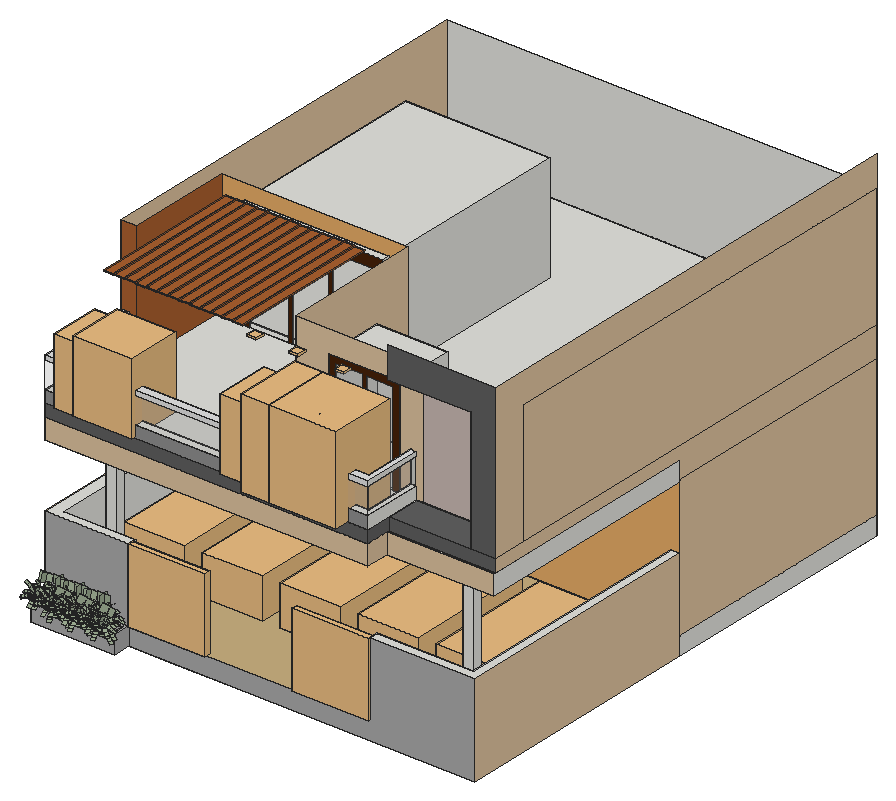
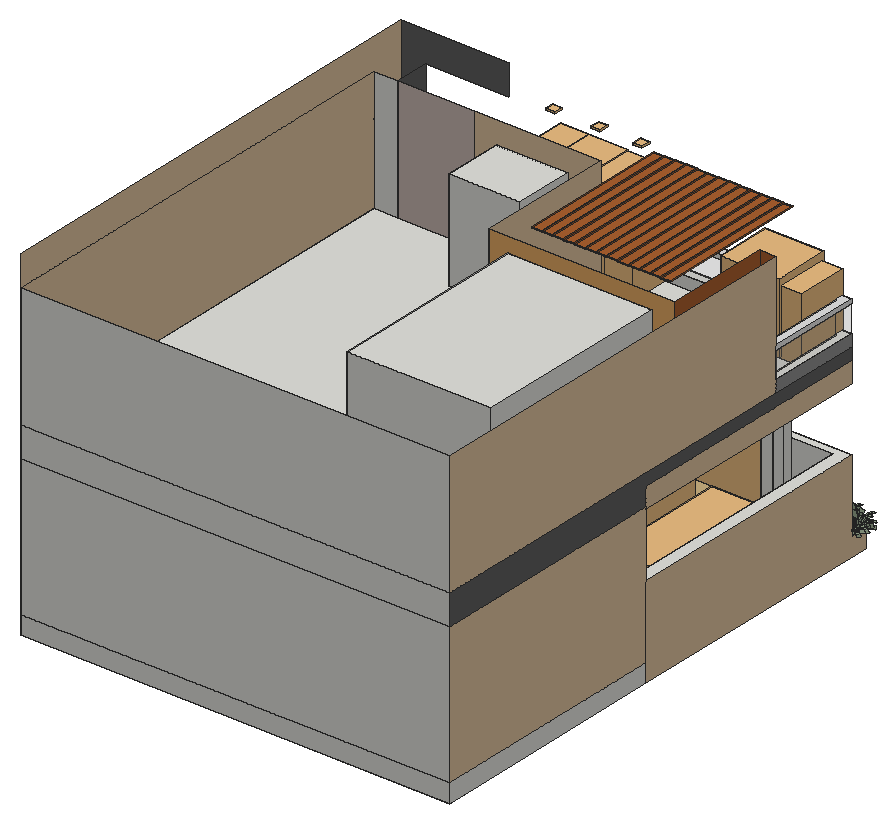
# SketchUp Ruby script. Lengths in inches.
U = 1.inch
M = Sketchup.active_model
def pt(a) = Geom::Point3d.new(a.map { |v| v * U })
def face(e, loops, mat)
  f = e.add_face(loops[0].map { |a| pt(a) })
  loops[1..].each { |l| e.add_face(l.map { |a| pt(a) }).erase! }
  f.material = f.back_material = mat if mat
  f
end
# faces: each face lists its corners as indices into pts; further lists are holes
def faces(e, pts, list, mat = nil) = list.each { |f| face(e, (f[0].is_a?(Array) ? f : [f]).map { |l| l.map { |i| pts[i] } }, mat) }
# xy, xz, yz: faces in a plane at the given z, y or x. An outline is a flat list of corners, or four numbers for a rectangle; further outlines are holes
def ring(l) = l.size == 4 ? [[l[0], l[1]], [l[2], l[1]], [l[2], l[3]], [l[0], l[3]]] : l.each_slice(2).to_a
def flat(e, list, mat, &to3) = list.each { |f| face(e, (f[0].is_a?(Array) ? f : [f]).map { |l| ring(l).map { |u, v| to3.(u, v) } }, mat) }
def xy(e, z, list, mat = nil) = flat(e, list, mat) { |x, y| [x, y, z] }
def xz(e, y, list, mat = nil) = flat(e, list, mat) { |x, z| [x, y, z] }
def yz(e, x, list, mat = nil) = flat(e, list, mat) { |y, z| [x, y, z] }
def lines(e, pts, list) = list.each { |a, b| e.add_line(pt(pts[a]), pt(pts[b])) }
# prism: a flat outline (further loops are holes) pulled along v
def prism(e, loops, v, mat = nil)
  f = face(e, loops, mat); d = Geom::Vector3d.new(v.map { |x| x * U })
  f.pushpull(f.normal.samedirection?(d) ? d.length : -d.length)
end
def box(e, o, s, mat = nil) = prism(e, [[o, [o[0] + s[0], o[1], o[2]], [o[0] + s[0], o[1] + s[1], o[2]], [o[0], o[1] + s[1], o[2]]]], [0, 0, s[2]], mat)
def at(x, y, z, deg = 0) = Geom::Transformation.translation(pt([x, y, z])) * Geom::Transformation.rotation(ORIGIN, Z_AXIS, deg.degrees)
def axes(o, x, y, z) = Geom::Transformation.new([*x, 0, *y, 0, *z, 0, *pt(o).to_a, 1])
def part(name) = M.definitions.add(name)
# library, detail: a bought-in or finely detailed component or shape, given as its bounding box
def library(name, o, s) = part(name).tap { |d| box(d.entities, o, s) }
def detail(e, o, s) = box(e.add_group.entities, o, s)
def put(e, d, t, mat = nil) = e.add_instance(d, t).tap { |i| i.material = mat if mat }
def group(e, t, mat = nil) = e.add_group.tap { |g| g.transformation = t; g.material = mat if mat }.entities
root = M.entities
M.materials.add("Generic").color = [222, 194, 159]
M.materials.add("Generic\#1").color = [230, 172, 103]
M.materials.add("Generic\#2").color = [241, 212, 157]
M.materials.add("[Color M01]").color = [226, 226, 226]
M.materials.add("[Color M03]").color = [170, 170, 170]
M.materials.add("[Color M04]").color = [142, 142, 142]
M.materials.add("[Color M07]").color = [96, 96, 96]
M.materials.add("[Roofing Slate Tan]").color = [200, 175, 128]
M.materials.add("[Stone Marble]").color = [201, 185, 179]
M.materials.add("[Translucent Glass Gray]").color = [175, 175, 175]
M.materials["[Translucent Glass Gray]"].alpha = 0.14
M.materials.add("[Wood Cherry Original]").color = [170, 96, 47]
M.materials.add("[Wood Veneer 01]").color = [71, 34, 9]
M.materials.add("hymenocallis littoralis").color = [156, 172, 146]
c1 = part("Group\#856")
xy(c1.entities,7.38,[[0,0,5.5,15.91]],"hymenocallis littoralis")
p = [[5.5,28.78,0],[5.5,26.79,3.44],[0,26.79,3.44],[0,28.78,0],[0,23.75,6],[5.5,23.75,6],
  [0,15.91,7.38],[5.5,15.91,7.38]]
faces(c1.entities,p,[[0,1,2,3],[4,2,1,5],[6,4,5,7]],"hymenocallis littoralis")
c2 = part("Group\#854")
xy(c2.entities,7.38,[[0,0,5.5,15.91],[0,15.91,5.5,23.87]],"hymenocallis littoralis")
p = [[5.5,31.07,4.3],[5.5,27.74,6.47],[0,27.74,6.47],[0,31.07,4.3],[0,23.87,7.38],[5.5,23.87,7.38]]
faces(c2.entities,p,[[0,1,2,3],[4,2,1,5]],"hymenocallis littoralis")
c3 = part("Group\#857")
xy(c3.entities,7.38,[[0,0,5.6,15.91]],"hymenocallis littoralis")
p = [[5.6,28.78,0],[5.6,26.79,3.44],[0,26.79,3.44],[0,28.78,0],[0,23.75,6],[5.6,23.75,6],
  [0,15.91,7.38],[5.6,15.91,7.38]]
faces(c3.entities,p,[[0,1,2,3],[4,2,1,5],[6,4,5,7]],"hymenocallis littoralis")
c4 = part("Group\#855")
put(c4.entities,c2,axes([6.09,8.57,-0.52],[0.446,0.85617,0.26089],[-0.18444,-0.19731,0.96283],[0.87582,-0.47754,0.0699]))
put(c4.entities,c2,axes([6.29,7.28,-1.71],[0.37058,0.92707,-0.05667],[-0.32382,0.19004,0.99128],[0.87712,-0.32925,0.34964]))
put(c4.entities,c2,axes([11.04,16.14,-0.7],[1,0,0],[0,0.16628,1.02662],[0,-1.18456,0.19186]))
c5 = part("Group\#860")
put(c5.entities,c1,axes([24.57,32.05,-1.76],[0.9552,-0.22102,-0.19681],[0.4036,0.95545,0.88585],[-0.00568,-0.67859,0.7345]))
put(c5.entities,c1,axes([23.95,29.24,-2.4],[0,1,0],[-0.76041,0,0.64945],[0.64945,0,0.76041]))
put(c5.entities,c1,axes([24.22,24.72,-0.48],[-0.70711,0.70711,0],[-0.32757,-0.32757,0.80237],[0.61237,0.61237,0.5]))
put(c5.entities,c2,axes([20.66,37.22,-0.63],[1.12361,0.03262,0.39091],[-0.43499,0.29739,0.78777],[0.09852,-1.27434,0.37535]))
put(c5.entities,c1,axes([28.75,24.45,-2.4],[-1,0,0],[0,-0.76041,0.64945],[0,0.64945,0.76041]))
put(c5.entities,c3,axes([30.4,30.98,-3.7],[0.65676,-0.72002,0.22414],[0.55667,0.66341,0.5],[-0.50871,-0.20361,0.83652]))
put(c5.entities,c3,axes([32.41,29.61,-3.7],[0.04029,-0.97372,0.22414],[0.85287,0.15038,0.5],[-0.52057,0.17102,0.83652]))
put(c5.entities,c1,axes([31.89,25.85,-1.76],[-0.92056,0.33739,-0.19681],[-0.5186,-0.89824,0.88585],[0.08952,0.67268,0.7345]))
put(c5.entities,c1,axes([25.55,34.78,-0.48],[0.86603,0.5,0],[-0.25,0.43301,0.86603],[0.43301,-0.75,0.5]))
put(c5.entities,c3,axes([20.4,16.9375,-8.07],[-0.70711,0.70711,0],[-0.35754,-0.35754,0.65422],[1.3987,1.3987,1.52882]))
put(c5.entities,c1,axes([32.86,34.14,-0.48],[0.76604,-0.64279,0],[0.32139,0.38302,0.86603],[-0.55667,-0.66341,0.5]))
put(c5.entities,c1,axes([27.15,34.7,-0.1],[0.82472,-0.17528,-0.53769],[0.53769,0.53769,0.64945],[0.17528,-0.82472,0.53769]))
put(c5.entities,c1,axes([33.58,28.77,-2.4],[0,-1,0],[0.76041,0,0.64945],[-0.64945,0,0.76041]))
put(c5.entities,c1,axes([26.43,23.87,-2.81],[-0.75126,0.04415,0.65853],[0.53769,-0.53769,0.64945],[0.38276,0.84199,0.3802]))
put(c5.entities,c1,axes([28.78,23.98,-2.4],[-1,0,0],[0,-0.76041,0.64945],[0,0.64945,0.76041]))
put(c5.entities,c1,axes([25.39,25.38,-2.4],[-0.70711,0.70711,0],[-0.53769,-0.53769,0.64945],[0.45923,0.45923,0.76041]))
put(c5.entities,c1,axes([27.32,21.63,-0.1],[-0.45923,0.70711,-0.53769],[-0.76041,0,0.64945],[0.45923,0.70711,0.53769]))
put(c5.entities,c1,axes([25.17,27.625,-1.76],[0.56416,0.80187,-0.19681],[-0.66673,0.66673,0.80532],[0.62659,-0.26057,0.7345]))
put(c5.entities,c3,axes([27.59,27.04,-3.96],[-0.8993,-0.06127,0.43301],[0.2962,-0.8138,0.5],[0.32175,0.57791,0.75]))
put(c5.entities,c3,axes([26.98,24.5,-3.18],[-0.5,0.86603,0],[-0.75,-0.43301,0.5],[0.43301,0.25,0.86603]))
put(c5.entities,c3,axes([24.55,27.74,-3.7],[0.29517,0.92878,0.22414],[-0.85287,0.15038,0.5],[0.43068,-0.33875,0.83652]))
put(c5.entities,c3,axes([24.26,29.8,-3.18],[0.76604,0.64279,0],[-0.47317,0.5639,0.425],[0.32139,-0.38302,0.86603]))
put(c5.entities,c3,axes([25.98,32.46,-3.18],[1,0,0],[0,0.86603,0.5],[0,-0.5,0.86603]))
put(c5.entities,c1,axes([28.78,33.57,-2.4],[1,0,0],[0,0.76041,0.64945],[0,-0.64945,0.76041]))
put(c5.entities,c4,at(14.99,21.38,2.5))
put(c5.entities,c2,axes([34.63,26.34,-1.46],[-0.70089,-0.70877,0.07994],[0.4756,-0.38088,0.79293],[-0.53156,0.59378,0.60405]))
put(c5.entities,c2,axes([28.14,16.92,1.8125],[-1.19719,0.6912,0],[-0.09607,-0.16641,0.94244],[0.68444,1.18549,0.17613]))
put(c5.entities,c2,axes([31.5625,35.84,0.97],[0.66765,-1.1564,0.35779],[0.04445,0.30732,0.91033],[-1.20828,-0.64496,0.17012]))
put(c5.entities,c2,axes([38.94,22.51,0.89],[-0.97932,-0.67164,-0.05202],[0.27787,-0.41401,0.90999],[-0.85985,0.93577,0.32097]))
put(c5.entities,c2,axes([38.44,21.09,1.98],[-1.02864,-0.54856,0.2395],[0.33481,0.06999,0.88388],[-0.77261,1.08328,0.06417]))
put(c5.entities,c3,axes([35.02,30.51,-1.3],[-0.17365,-0.98481,0],[0.60224,-0.10619,0.79122],[-0.7792,0.13739,0.61153]))
put(c5.entities,c3,axes([29.41,22.33,-1.3],[-0.93969,0.34202,0],[-0.20915,-0.57465,0.79122],[0.27061,0.74351,0.61153]))
put(c5.entities,c2,axes([19.64,36,-1.62],[1.18194,0.09546,0.08234],[-0.14377,0.68823,0.76313],[0.21457,-1.1326,0.62386]))
put(c5.entities,c3,axes([24.25,24.14,-1.3],[-0.34202,0.93969,0],[-0.57465,-0.20915,0.79122],[0.74351,0.27061,0.61153]))
put(c5.entities,c3,axes([25.98,34.61,-1.3],[1,0,0],[0,0.61153,0.79122],[0,-0.79122,0.61153]))
put(c5.entities,c3,axes([31.16,34.41,-1.64],[0.56518,-0.80224,-0.19234],[0.73413,0.34233,0.72935],[-0.47639,-0.50772,0.71782]))
put(c5.entities,c3,axes([40.52,26.84,-5.82],[-0.42262,-0.90631,0],[0.48019,-0.22391,0.68552],[-1.43418,0.66877,1.22305]))
put(c5.entities,c1,axes([29.86,38.42,-1.01],[0.89064,-0.37013,0.26413],[-0.03924,0.63286,1.01918],[-0.45353,-0.76487,0.45748]))
put(c5.entities,c1,axes([29.34,22.4,-0.48],[-0.99619,-0.08716,0],[0.04358,-0.4981,0.86603],[-0.07548,0.86273,0.5]))
c6 = part("Group\#858")
xz(c6.entities,10.07,[[9.07,0,10.07,31.01],[0,31.01,0,45.12,20.13,45.12,20.13,31.01,10.07,31.01,10.07,32.58,9.07,32.58,9.07,31.01]],"hymenocallis littoralis")
yz(c6.entities,10.07,[[0,31.01,20.13,45.12]],"hymenocallis littoralis")
p = [[9.57,9.2,0],[10.07,10.07,0],[10.07,10.07,31.01],[10.07,10.07,32.58],[9.57,9.2,32.58]]
faces(c6.entities,p,[[0,1,2,3,4]],"hymenocallis littoralis")
c7 = part("cây lá nắng")
put(c7.entities,c5,axes([49.26,-2.75,0],[0.63109,0.63109,0],[-0.63109,0.63109,0],[0,0,0.935]))
g1 = group(c7.entities,at(26.6,-8.68,0))
put(g1,c1,axes([-4.72,35.73,-1.65],[0.74231,0.46334,-0.18402],[-0.34827,0.85768,0.82827],[0.42467,-0.43184,0.68675]))
put(g1,c1,axes([-3.34,33.57,-2.24],[-0.63109,0.63109,0],[-0.47989,-0.47989,0.60723],[0.40986,0.40986,0.71098]))
put(g1,c1,axes([-0.3125,30.89,-0.45],[-0.8925,0,0],[0,-0.41345,0.75022],[0,0.77293,0.4675]))
put(g1,c2,axes([-10.79,39.66,-0.59],[0.68852,0.72969,0.3655],[-0.4622,-0.08684,0.73657],[0.86641,-0.74205,0.35095]))
put(g1,c1,axes([2.71,33.57,-2.24],[-0.63109,-0.63109,0],[0.47989,-0.47989,0.60723],[-0.40986,0.40986,0.71098]))
put(g1,c3,axes([-0.37,38.74,-3.46],[0.86887,-0.03992,0.20957],[-0.06737,0.76999,0.4675],[-0.19255,-0.44954,0.78214]))
put(g1,c3,axes([1.76,39.14,-3.46],[0.63993,-0.58908,0.20957],[0.44333,0.63315,0.4675],[-0.43646,-0.2206,0.78214]))
put(g1,c1,axes([3.81,36.4375,-1.65],[-0.79389,-0.36803,-0.18402],[0.23959,-0.89415,0.82827],[-0.36803,0.48102,0.68675]))
put(g1,c1,axes([-5.83,38.07,-0.45],[0.231,0.86209,0],[-0.43104,0.1155,0.80973],[0.74659,-0.20005,0.4675]))
put(g1,c3,axes([2.18,23.5625,-7.55],[-0.8925,0,0],[0,-0.45128,0.6117],[0,1.76542,1.42944]))
put(g1,c1,axes([-0.8125,42.28,-0.45],[0.8891,0.07779,0],[-0.03889,0.44455,0.80973],[0.06737,-0.76999,0.4675]))
put(g1,c1,axes([-4.76,39.03,-0.09],[0.63109,0.40986,-0.50274],[0,0.67866,0.60723],[0.63109,-0.40986,0.50274]))
put(g1,c1,axes([3.03,39.35,-2.24],[0.63109,-0.63109,0],[0.47989,0.47989,0.60723],[-0.40986,-0.40986,0.71098]))
put(g1,c1,axes([1.61,31.74,-2.625],[-0.50198,-0.44625,0.61573],[0.67866,0,0.60723],[-0.28982,0.77293,0.35549]))
put(g1,c1,axes([3.03,33.3,-2.24],[-0.63109,-0.63109,0],[0.47989,-0.47989,0.60723],[-0.40986,0.40986,0.71098]))
put(g1,c1,axes([0.01,32.04,-2.24],[-0.8925,0,0],[0,-0.67866,0.60723],[0,0.57963,0.71098]))
put(g1,c1,axes([3.59,30.89,-0.09],[-0.73607,0.15643,-0.50274],[-0.47989,-0.47989,0.60723],[-0.15643,0.73607,0.50274]))
put(g1,c1,axes([-1.55,33.32,-1.65],[-0.15002,0.86209,-0.18402],[-0.84154,0,0.75297],[0.55988,0.231,0.68675]))
put(g1,c3,axes([0.35,34.48,-3.71],[-0.52887,-0.60621,0.40487],[0.70051,-0.32665,0.4675],[-0.16166,0.56777,0.70125]))
put(g1,c3,axes([2.61,39.13,-1.74],[-0.86209,0.231,0],[-0.23031,-0.85954,0.15531],[0.03162,0.11799,0.91645]))
put(g1,c3,axes([-2.02,33,-3.46],[-0.39986,0.77243,0.20957],[-0.63315,-0.44333,0.4675],[0.48558,0.05802,0.78214]))
put(g1,c3,axes([-3.49,34.12,-2.97],[0.07779,0.8891,0],[-0.65449,0.05726,0.39737],[0.44455,-0.03889,0.80973]))
put(g1,c3,axes([-4.09,36.88,-2.97],[0.63109,0.63109,0],[-0.54654,0.54654,0.4675],[0.31555,-0.31555,0.80973]))
put(g1,c1,axes([-3.02,39.35,-2.24],[0.63109,0.63109,0],[-0.47989,0.47989,0.60723],[0.40986,-0.40986,0.71098]))
put(g1,c4,axes([-4.03,22.95,2.33],[0.63109,0.63109,0],[-0.63109,0.63109,0],[0,0,0.935]))
put(g1,c2,axes([5.24,38.48,-1.37],[0.00497,-0.88963,0.07474],[0.54052,0.05978,0.74139],[-0.71019,0.03927,0.56479]))
put(g1,c2,axes([7.08,28.4375,1.7],[-1.19175,-0.31933,0],[0.04439,-0.16565,0.88118],[-0.31621,1.1801,0.16468]))
put(g1,c2,axes([-2.7,42.54,0.91],[1.15114,-0.30845,0.33454],[-0.1659,0.22199,0.85115],[-0.3555,-1.16957,0.15907]))
put(g1,c2,axes([10.37,38.78,0.83],[-0.19417,-1.04191,-0.04864],[0.43664,-0.08592,0.85084],[-1.1332,0.04791,0.30011]))
put(g1,c2,axes([10.95,37.5625,1.85],[-0.30298,-0.99536,0.22393],[0.16713,0.25547,0.82643],[-1.17124,0.19607,0.06]))
put(g1,c3,axes([2.84,41.36,-1.22],[0.51192,-0.73109,0],[0.44708,0.31305,0.73979],[-0.57846,-0.40504,0.57178]))
put(g1,c3,axes([4.47,32.65,-1.22],[-0.80888,-0.37719,0],[0.23066,-0.49465,0.73979],[-0.29844,0.64,0.57178]))
put(g1,c2,axes([-10.32,35.12,-1.51],[0.68567,0.80616,0.07699],[-0.52507,0.3436,0.71352],[0.85019,-0.57936,0.58331]))
put(g1,c3,axes([0.07,30.54,-1.22],[-0.80888,0.37719,0],[-0.23066,-0.49465,0.73979],[0.29844,0.64,0.57178]))
put(g1,c3,axes([-5.45,38.24,-1.22],[0.63109,0.63109,0],[-0.38593,0.38593,0.73979],[0.49934,-0.49934,0.57178]))
put(g1,c3,axes([-2.05,41.38,-1.53],[0.86296,-0.14961,-0.17984],[0.24726,0.67935,0.68194],[0.01977,-0.62107,0.67116]))
put(g1,c3,axes([8.63,42.51,-5.4375],[0.30525,-0.83868,0],[0.44435,0.16173,0.64096],[-1.32716,-0.48305,1.14356]))
put(g1,c1,axes([-5.4,43.09,-0.94],[0.79566,0.32849,0.24696],[-0.42416,0.37462,0.95293],[0.19648,-0.76892,0.42774]))
put(g1,c1,axes([4.38,32.65,-0.45],[-0.57369,-0.68369,0],[0.34185,-0.28684,0.80973],[-0.5921,0.49683,0.4675]))
put(g1,c3,axes([-2,33.84,-0.15],[-0.24601,0.85793,0],[-0.85539,-0.24528,0.15531],[0.11742,0.03367,0.91645]))
put(g1,c3,axes([0.17,30.83,-4.47],[-0.24601,0.85793,0],[-0.85539,-0.24528,0.15531],[0.11742,0.03367,0.91645]))
put(g1,c3,axes([-1.97,32.18,-4.47],[0.58524,0.67383,0],[-0.67184,0.58351,0.15531],[0.09222,-0.0801,0.91645]))
put(g1,c3,axes([-2,34.71,-4.47],[0.88392,-0.12346,0],[0.12309,0.88131,0.15531],[-0.0169,-0.12098,0.91645]))
put(g1,c3,axes([0.11,36.12,-4.47],[0.37822,-0.8084,0],[0.80601,0.37711,0.15531],[-0.11064,-0.05177,0.91645]))
put(c7.entities,c6,axes([29.71,14.29,6.94],[0.425,0.73612,0],[-0.6771,0.39092,-0.33349],[-0.26859,0.15507,0.72712]))
put(c7.entities,c6,axes([42.0625,26.12,6.94],[0.85,0,0],[0,0.78185,-0.33349],[0,0.33349,0.78185]))
put(c7.entities,c5,axes([7.3125,23.0625,0],[0.8925,0,0],[0,0.8925,0],[0,0,0.935]))
put(c7.entities,c6,axes([24.4375,40.23,2.05],[0.85,0,0],[0,0.85,0],[0,0,0.85]))
c8 = part("Planting+101")
put(c8.entities,c7,axes([21.34,32.96,-4.59],[0,-0.71,0],[-0.71,0,0],[0,0,0.71]))
c9 = library("Group\#6",[0,0,0],[126.8125,5.75,72.25])
c10 = library("2016+Honda+Civic+LX+Sedan",[0.01,0.03,0.02],[16.17,34.46,10.62])
c11 = library("Tlon Light 450 Ceiling 152 006",[-8.86,-8.86,-3.78],[17.72,17.72,3.56])
c12 = library("Plant+2 (1)",[-9.13,-9.52,0],[51.76,51.77,66.88])
c13 = library("Plante 4",[-1.67,-6.5,0],[37.31,31.95,64.42])
c14 = part("Group\#3")
xy(c14.entities,0,[[0,0,140.875,6.8125]])
xy(c14.entities,105.3125,[[0,0,140.875,6.8125]])
xz(c14.entities,0,[[10.8,0,48.56,94.52],[52.56,0,88.32,94.52],[92.32,0,130.08,94.52]],"[Translucent Glass Gray]")
xz(c14.entities,0,[[0,0,10.8,0,10.8,94.52,48.56,94.52,48.56,0,52.56,0,52.56,94.52,88.32,94.52,88.32,0,92.32,0,92.32,94.52,130.08,94.52,130.08,0,140.875,0,140.875,105.3125,0,105.3125]],"[Wood Veneer 01]")
xz(c14.entities,6.8125,[[0,0,140.875,105.3125]],"[Translucent Glass Gray]")
yz(c14.entities,0,[[0,0,6.8125,105.3125]])
yz(c14.entities,140.875,[[0,0,6.8125,105.3125]])
c15 = library("Group3\#1",[-238.15,54.18,0],[46.4,43.96,56.68])
xy(root,-34.4375,[[20.1875,14.66,20.1875,283.54,132.9375,283.54,132.9375,32.23,102.3125,32.23,102.3125,14.66],[132.9375,32.23,234.5,113.91],[234.5,32.23,440.1875,283.54],[132.9375,113.91,234.5,365.23],[20.1875,283.54,20.1875,523.73,440.1875,523.73,440.1875,283.54,234.5,283.54,234.5,365.23,132.9375,365.23,132.9375,283.54]])
xy(root,-24.875,[[23.375,17.85,99.125,29.04]],"[Color M03]")
xy(root,-16.6875,[[20.1875,283.54,132.9375,283.54,132.9375,365.23,234.5,365.23,234.5,283.54,440.1875,283.54,440.1875,523.73,20.1875,523.73]])
xy(root,-16.6875,[[[20.1875,14.66,102.3125,32.23],[23.375,17.85,99.125,29.04]]],"[Color M03]")
xy(root,-16.6875,[[[102.3125,32.23,337.5,32.23,337.5,41.48,431.6875,41.48,431.6875,283.54,234.5,283.54,234.5,365.23,132.9375,365.23,132.9375,283.54,32.3125,283.54,32.3125,40.48,102.3125,40.48],[41.96,79.19,52.84,87.88],[390.96,79.19,401.84,87.88]]],"[Roofing Slate Tan]")
xy(root,55.5625,[[20.1875,32.23,102.3125,32.23,102.3125,40.48,32.3125,40.48,32.3125,283.54,20.1875,283.54],[337.5,32.23,440.1875,32.23,440.1875,283.54,431.6875,283.54,431.6875,41.48,337.5,41.48]])
xy(root,117.8125,[[20.1875,32.23,20.1875,283.54,132.9375,283.54,132.9375,365.23,234.5,365.23,234.5,283.54,440.1875,283.54,440.1875,55.6,335.49,55.6,335.49,32.23]],"Generic\#2")
xy(root,120,[[20.1875,283.54,20.1875,523.73,440.1875,523.73,440.1875,283.54,234.5,283.54,234.5,365.23,132.9375,365.23,132.9375,283.54]])
xy(root,137.6875,[[[20.1875,32.23,335.49,32.23,335.49,57.98,440.1875,57.98,440.1875,283.54,234.5,283.54,234.5,365.23,132.9375,365.23,132.9375,283.54,20.1875,283.54],[390.96,79.19,401.84,87.88]],[335.49,55.6,440.1875,57.98]])
xy(root,145.9375,[[41.96,79.19,52.84,87.88]])
xy(root,149.9375,[[20.1875,32.23,20.1875,125.1,28.125,125.1,28.125,40.98,329.87,40.98,329.87,91.73,335.49,91.73,335.49,32.23],[28.125,40.98,329.87,40.98,329.87,91.73,319.875,91.73,319.875,150.04,250.24,150.04,250.24,91.73,217.875,91.73,217.875,228.48,35.6875,228.48,35.6875,125.1,28.125,125.1],[335.49,57.98,336.74,91.73],[416.1875,57.98,440.1875,91.73],[217.875,91.73,217.875,228.48,35.6875,228.48,35.6875,125.1,20.1875,125.1,20.1875,523.73,440.1875,523.73,440.1875,91.73,319.875,91.73,319.875,150.04,250.24,150.04,250.24,91.73]])
xy(root,149.9375,[[336.74,57.98,416.1875,91.73]],"[Color M07]")
xy(root,150.0625,[[58.21,228.48,199.08,425.29]])
xy(root,161.4375,[[20.1875,32.23,20.1875,125.1,28.125,125.1,28.125,40.98,329.87,40.98,329.87,91.73,335.49,91.73,335.49,32.23]])
xy(root,187.4375,[[20.1875,32.23,20.1875,125.1,28.125,125.1,28.125,40.98,329.87,40.98,329.87,91.73,335.49,91.73,335.49,32.23]])
xy(root,192.125,[[20.1875,32.23,335.49,32.23,335.49,91.73,329.87,91.73,329.87,40.98,28.125,40.98,28.125,125.1,20.1875,125.1]],"[Color M01]")
xy(root,248.12,[[250.24,91.73,319.875,150.04]])
xy(root,255.375,[[58.21,228.48,199.08,425.29]])
xy(root,269.0625,[[58.88,55.42,67.93,205.29],[68.93,55.42,78.5,205.29],[79.5,55.42,89.06,205.29],[90.06,55.42,99.62,205.29],[100.62,55.42,110.18,205.29],
  [111.18,55.42,120.75,205.29],[121.75,55.42,131.31,205.29],[132.31,55.42,141.87,205.29],[142.87,55.42,152.43,205.29],[153.43,55.42,163,205.29],
  [164,55.42,173.56,205.29],[174.56,55.42,184.12,205.29],[185.12,55.42,194.68,205.29]],"[Wood Cherry Original]")
xz(root,14.66,[[20.1875,-34.4375,102.3125,-16.6875]],"[Color M03]")
xz(root,17.85,[[23.375,-24.875,99.125,-16.6875]],"[Color M03]")
xz(root,29.04,[[23.375,-24.875,99.125,-16.6875]],"[Color M03]")
xz(root,32.23,[[20.1875,117.8125,335.49,137.6875]],"Generic")
xz(root,32.23,[[20.1875,187.4375,335.49,192.125]],"[Color M01]")
xz(root,32.23,[[102.3125,-34.4375,440.1875,-34.4375,440.1875,55.5625,337.5,55.5625,337.5,-16.6875,102.3125,-16.6875],[20.1875,-16.6875,102.3125,55.5625]],"[Color M03]")
xz(root,32.23,[[20.1875,149.9375,335.49,161.4375]],"[Color M04]")
xz(root,32.23,[[20.1875,137.6875,335.49,149.9375]],"[Color M07]")
xz(root,32.23,[[20.1875,161.4375,335.49,187.4375]],"[Translucent Glass Gray]")
xz(root,40.48,[[32.3125,-16.6875,102.3125,55.5625]])
xz(root,40.98,[[28.125,149.9375,329.87,161.4375],[28.125,187.4375,329.87,192.125]])
xz(root,40.98,[[28.125,161.4375,329.87,187.4375]],"[Translucent Glass Gray]")
xz(root,41.48,[[337.5,-16.6875,431.6875,55.5625]])
xz(root,55.42,[[58.88,269.0625,67.93,269.9375],[68.93,269.0625,78.5,269.9375],[79.5,269.0625,89.06,269.9375],[90.06,269.0625,99.62,269.9375],[100.62,269.0625,110.18,269.9375],
  [111.18,269.0625,120.75,269.9375],[121.75,269.0625,131.31,269.9375],[132.31,269.0625,141.87,269.9375],[142.87,269.0625,152.43,269.9375],[153.43,269.0625,163,269.9375],
  [164,269.0625,173.56,269.9375],[174.56,269.0625,184.12,269.9375],[185.12,269.0625,194.68,269.9375]],"[Wood Cherry Original]")
xz(root,55.6,[[335.49,117.8125,440.1875,137.6875]],"Generic")
xz(root,57.98,[[335.49,137.6875,440.1875,149.9375],[416.1875,149.9375,440.1875,149.9375,440.1875,299.875,335.12,299.875,335.12,269.9375,416.1875,269.9375]],"[Color M07]")
xz(root,79.19,[[41.96,-16.6875,52.84,145.9375],[390.96,-16.6875,401.84,137.6875]])
xz(root,87.88,[[41.96,-16.6875,52.84,145.9375],[390.96,-16.6875,401.84,137.6875]])
xz(root,91.73,[[416.1875,149.9375,440.1875,269.9375]])
xz(root,91.73,[[217.875,149.9375,250.24,149.9375,250.24,248.12,319.875,248.12,319.875,149.9375,329.87,149.9375,329.87,192.125,335.49,192.125,335.49,149.9375,342.11,149.9375,342.11,269.9375,217.875,269.9375]],"Generic")
xz(root,91.73,[[342.11,149.9375,416.1875,269.9375]],"[Stone Marble]")
xz(root,125.1,[[28.125,149.9375,35.6875,149.9375,35.6875,269.9375,20.1875,269.9375,20.1875,192.125,28.125,192.125]],"[Wood Cherry Original]")
xz(root,150.04,[[250.24,149.9375,319.875,248.12]])
xz(root,205.29,[[58.88,269.0625,67.93,269.9375],[68.93,269.0625,78.5,269.9375],[79.5,269.0625,89.06,269.9375],[90.06,269.0625,99.62,269.9375],[100.62,269.0625,110.18,269.9375],
  [111.18,269.0625,120.75,269.9375],[121.75,269.0625,131.31,269.9375],[132.31,269.0625,141.87,269.9375],[142.87,269.0625,152.43,269.9375],[153.43,269.0625,163,269.9375],
  [164,269.0625,173.56,269.9375],[174.56,269.0625,184.12,269.9375],[185.12,269.0625,194.68,269.9375]])
xz(root,228.48,[[[35.6875,149.9375,217.875,269.9375],[58.21,150.0625,199.08,255.375]]],"Generic\#1")
xz(root,283.54,[[20.1875,-34.4375,132.9375,-16.6875],[234.5,-34.4375,440.1875,-16.6875],[20.1875,-16.6875,32.3125,55.5625],[20.1875,117.8125,132.9375,120],[234.5,117.8125,440.1875,120],
  [20.1875,120,132.9375,137.6875],[234.5,120,440.1875,137.6875]])
xz(root,283.54,[[32.3125,-16.6875,132.9375,-16.6875,132.9375,117.8125,20.1875,117.8125,20.1875,55.5625,32.3125,55.5625]],"Generic")
xz(root,283.54,[[234.5,-16.6875,431.6875,-16.6875,431.6875,55.5625,440.1875,55.5625,440.1875,117.8125,234.5,117.8125]],"Generic\#1")
xz(root,365.23,[[132.9375,-34.4375,234.5,-16.6875],[132.9375,117.8125,234.5,120],[132.9375,120,234.5,137.6875]])
xz(root,365.23,[[132.9375,-16.6875,234.5,117.8125]],"[Wood Cherry Original]")
xz(root,425.29,[[58.21,150.0625,199.08,255.375]])
xz(root,523.73,[[20.1875,-34.4375,440.1875,-16.6875],[20.1875,-16.6875,440.1875,120],[20.1875,120,440.1875,149.9375],[20.1875,149.9375,440.1875,269.9375]])
yz(root,20.1875,[[283.54,-34.4375,523.73,-16.6875]])
yz(root,20.1875,[[14.66,-34.4375,14.66,-16.6875,32.23,-16.6875,32.23,55.5625,283.54,55.5625,283.54,-34.4375],[283.54,-16.6875,523.73,120],[32.23,117.8125,283.54,137.6875],[125.1,149.9375,523.73,269.9375]],"Generic")
yz(root,20.1875,[[32.23,187.4375,125.1,192.125]],"[Color M01]")
yz(root,20.1875,[[32.23,149.9375,125.1,161.4375]],"[Color M04]")
yz(root,20.1875,[[283.54,120,283.54,137.6875,32.23,137.6875,32.23,149.9375,523.73,149.9375,523.73,120]],"[Color M07]")
yz(root,20.1875,[[32.23,161.4375,125.1,187.4375]],"[Translucent Glass Gray]")
yz(root,23.375,[[17.85,-24.875,29.04,-16.6875]],"[Color M03]")
yz(root,28.125,[[40.98,149.9375,125.1,161.4375],[40.98,187.4375,125.1,192.125]])
yz(root,28.125,[[40.98,161.4375,125.1,187.4375]],"[Translucent Glass Gray]")
yz(root,32.3125,[[40.48,-16.6875,283.54,55.5625]])
yz(root,35.6875,[[125.1,149.9375,228.48,269.9375]],"[Wood Cherry Original]")
yz(root,41.96,[[79.19,-16.6875,87.88,145.9375]])
yz(root,52.84,[[79.19,-16.6875,87.88,145.9375]])
yz(root,58.21,[[228.48,150.0625,425.29,255.375]])
yz(root,58.88,[[55.42,269.0625,101.91,269.9375],[101.91,269.0625,205.29,269.9375]],"[Wood Cherry Original]")
yz(root,67.93,[[55.42,269.0625,68.54,269.9375],[68.54,269.0625,205.29,269.9375]],"[Wood Cherry Original]")
yz(root,68.93,[[55.42,269.0625,68.54,269.9375],[68.54,269.0625,205.29,269.9375]],"[Wood Cherry Original]")
yz(root,78.5,[[55.42,269.0625,68.54,269.9375],[68.54,269.0625,205.29,269.9375]],"[Wood Cherry Original]")
yz(root,79.5,[[55.42,269.0625,68.54,269.9375],[68.54,269.0625,205.29,269.9375]],"[Wood Cherry Original]")
yz(root,89.06,[[55.42,269.0625,68.54,269.9375],[68.54,269.0625,205.29,269.9375]],"[Wood Cherry Original]")
yz(root,90.06,[[55.42,269.0625,68.54,269.9375],[68.54,269.0625,205.29,269.9375]],"[Wood Cherry Original]")
yz(root,99.125,[[17.85,-24.875,29.04,-16.6875]],"[Color M03]")
yz(root,99.62,[[55.42,269.0625,68.54,269.9375],[68.54,269.0625,205.29,269.9375]],"[Wood Cherry Original]")
yz(root,100.62,[[55.42,269.0625,68.54,269.9375],[68.54,269.0625,205.29,269.9375]],"[Wood Cherry Original]")
yz(root,102.3125,[[32.23,-16.6875,40.48,55.5625]])
yz(root,102.3125,[[14.66,-34.4375,32.23,-16.6875]],"[Color M03]")
yz(root,110.18,[[55.42,269.0625,68.54,269.9375],[68.54,269.0625,205.29,269.9375]],"[Wood Cherry Original]")
yz(root,111.18,[[55.42,269.0625,68.54,269.9375],[68.54,269.0625,205.29,269.9375]],"[Wood Cherry Original]")
yz(root,120.75,[[55.42,269.0625,68.54,269.9375],[68.54,269.0625,205.29,269.9375]],"[Wood Cherry Original]")
yz(root,121.75,[[55.42,269.0625,68.54,269.9375],[68.54,269.0625,205.29,269.9375]],"[Wood Cherry Original]")
yz(root,131.31,[[55.42,269.0625,68.54,269.9375],[68.54,269.0625,205.29,269.9375]],"[Wood Cherry Original]")
yz(root,132.31,[[55.42,269.0625,68.54,269.9375],[68.54,269.0625,205.29,269.9375]],"[Wood Cherry Original]")
yz(root,132.9375,[[283.54,-34.4375,365.23,-16.6875],[283.54,117.8125,365.23,120],[283.54,120,365.23,137.6875]])
yz(root,132.9375,[[283.54,-16.6875,365.23,117.8125]],"[Wood Cherry Original]")
yz(root,141.87,[[55.42,269.0625,68.54,269.9375],[68.54,269.0625,205.29,269.9375]],"[Wood Cherry Original]")
yz(root,142.87,[[55.42,269.0625,68.54,269.9375],[68.54,269.0625,205.29,269.9375]],"[Wood Cherry Original]")
yz(root,152.43,[[55.42,269.0625,68.54,269.9375],[68.54,269.0625,205.29,269.9375]],"[Wood Cherry Original]")
yz(root,153.43,[[55.42,269.0625,68.54,269.9375],[68.54,269.0625,205.29,269.9375]],"[Wood Cherry Original]")
yz(root,163,[[55.42,269.0625,68.54,269.9375],[68.54,269.0625,205.29,269.9375]],"[Wood Cherry Original]")
yz(root,164,[[55.42,269.0625,68.54,269.9375],[68.54,269.0625,205.29,269.9375]],"[Wood Cherry Original]")
yz(root,173.56,[[55.42,269.0625,68.54,269.9375],[68.54,269.0625,205.29,269.9375]],"[Wood Cherry Original]")
yz(root,174.56,[[55.42,269.0625,68.54,269.9375],[68.54,269.0625,205.29,269.9375]],"[Wood Cherry Original]")
yz(root,184.12,[[55.42,269.0625,68.54,269.9375],[68.54,269.0625,205.29,269.9375]],"[Wood Cherry Original]")
yz(root,185.12,[[55.42,269.0625,68.54,269.9375],[68.54,269.0625,205.29,269.9375]],"[Wood Cherry Original]")
yz(root,194.68,[[55.42,269.0625,68.54,269.9375],[68.54,269.0625,205.29,269.9375]],"[Wood Cherry Original]")
yz(root,199.08,[[228.48,150.0625,425.29,255.375]])
yz(root,217.875,[[91.73,149.9375,228.48,269.9375]],"Generic")
yz(root,234.5,[[283.54,-34.4375,365.23,-16.6875],[283.54,117.8125,365.23,120],[283.54,120,365.23,137.6875]])
yz(root,234.5,[[283.54,-16.6875,365.23,117.8125]],"[Wood Cherry Original]")
yz(root,250.24,[[91.73,149.9375,150.04,248.12]])
yz(root,319.875,[[91.73,149.9375,150.04,248.12]])
yz(root,329.87,[[40.98,149.9375,91.73,161.4375],[40.98,187.4375,91.73,192.125]])
yz(root,329.87,[[40.98,161.4375,91.73,187.4375]],"[Translucent Glass Gray]")
yz(root,335.49,[[32.23,149.9375,91.73,161.4375],[32.23,187.4375,91.73,192.125]])
yz(root,335.49,[[32.23,117.8125,55.6,137.6875]],"Generic")
yz(root,335.49,[[32.23,137.6875,57.98,149.9375]],"[Color M07]")
yz(root,335.49,[[32.23,161.4375,91.73,187.4375]],"[Translucent Glass Gray]")
yz(root,337.5,[[32.23,-16.6875,41.48,55.5625]])
yz(root,390.96,[[79.19,-16.6875,87.88,137.6875]])
yz(root,401.84,[[79.19,-16.6875,87.88,137.6875]])
yz(root,416.1875,[[57.98,149.9375,91.73,269.9375]],"[Color M07]")
yz(root,431.6875,[[41.48,-16.6875,283.54,55.5625]])
yz(root,440.1875,[[283.54,-34.4375,523.73,-16.6875],[55.6,117.8125,283.54,137.6875]])
yz(root,440.1875,[[32.23,-34.4375,283.54,55.5625],[283.54,-16.6875,523.73,120],[283.54,120,523.73,120,523.73,149.9375,57.98,149.9375,57.98,137.6875,283.54,137.6875],[57.98,149.9375,91.73,149.9375,91.73,269.9375,523.73,269.9375,523.73,299.875,57.98,299.875],[91.73,149.9375,523.73,269.9375]],"Generic")
p = [[335.49,32.23,117.8125],[335.49,32.23,116.75],[234.5,113.91,-16.6875],[234.5,113.91,-34.4375]]
lines(root,p,[[0,1],[2,3]])
put(root,c8,axes([27.84,17.51,-18.0625],[0,-0.82091,0],[1,0,0],[0,0,1]))
put(root,c8,axes([48.84,17.51,-18.0625],[0,-0.82091,0],[1,0,0],[0,0,1]))
put(root,c8,axes([71.15,17.51,-18.0625],[0,-0.82091,0],[1,0,0],[0,0,1]))
put(root,c9,axes([102.3125,31.23,-16.6875],[0.5916,0,0],[0,1,0],[0,0,1]))
put(root,c9,axes([262.48,31.23,-16.6875],[0.5916,0,0],[0,1,0],[0,0,1]))
put(root,c10,axes([45.55,96.78,-12.74],[3.67104,0,0],[0,3.67104,0],[0,0,3.67104]))
put(root,c10,axes([121.92,96.78,-12.74],[3.67104,0,0],[0,3.67104,0],[0,0,3.67104]))
put(root,c10,axes([198.3,96.78,-12.74],[3.67104,0,0],[0,3.67104,0],[0,0,3.67104]))
put(root,c10,axes([274.67,96.78,-12.74],[3.67104,0,0],[0,3.67104,0],[0,0,3.67104]))
put(root,c10,axes([351.05,96.78,-12.74],[3.67104,0,0],[0,3.67104,0],[0,0,3.67104]))
put(root,c11,axes([75.62,84.54,117.92],[0.5,0,0],[0,0.5,0],[0,0,0.5]))
put(root,c11,axes([75.62,125.79,117.92],[0.5,0,0],[0,0.5,0],[0,0,0.5]))
put(root,c11,axes([75.62,167.04,117.92],[0.5,0,0],[0,0.5,0],[0,0,0.5]))
put(root,c11,axes([75.62,208.29,117.92],[0.5,0,0],[0,0.5,0],[0,0,0.5]))
put(root,c11,axes([147.5,88.29,117.92],[0.5,0,0],[0,0.5,0],[0,0,0.5]))
put(root,c11,axes([147.5,129.54,117.92],[0.5,0,0],[0,0.5,0],[0,0,0.5]))
put(root,c11,axes([147.5,212.04,117.92],[0.5,0,0],[0,0.5,0],[0,0,0.5]))
put(root,c11,axes([147.5,170.79,117.92],[0.5,0,0],[0,0.5,0],[0,0,0.5]))
put(root,c11,axes([375.9,148.5,117.92],[0.5,0,0],[0,0.5,0],[0,0,0.5]))
put(root,c11,axes([375.9,231,117.92],[0.5,0,0],[0,0.5,0],[0,0,0.5]))
put(root,c11,axes([375.9,189.75,117.92],[0.5,0,0],[0,0.5,0],[0,0,0.5]))
put(root,c11,axes([375.9,107.25,117.92],[0.5,0,0],[0,0.5,0],[0,0,0.5]))
put(root,c11,axes([325.15,91.69,117.92],[0.5,0,0],[0,0.5,0],[0,0,0.5]))
put(root,c11,axes([325.15,132.94,117.92],[0.5,0,0],[0,0.5,0],[0,0,0.5]))
put(root,c11,axes([325.15,215.44,117.92],[0.5,0,0],[0,0.5,0],[0,0,0.5]))
put(root,c11,axes([325.15,174.19,117.92],[0.5,0,0],[0,0.5,0],[0,0,0.5]))
put(root,c11,axes([276.8125,79.9,117.92],[0.5,0,0],[0,0.5,0],[0,0,0.5]))
put(root,c11,axes([276.8125,121.15,117.92],[0.5,0,0],[0,0.5,0],[0,0,0.5]))
put(root,c11,axes([276.8125,203.65,117.92],[0.5,0,0],[0,0.5,0],[0,0,0.5]))
put(root,c11,axes([276.8125,162.4,117.92],[0.5,0,0],[0,0.5,0],[0,0,0.5]))
put(root,c11,axes([228.48,79.61,117.92],[0.5,0,0],[0,0.5,0],[0,0,0.5]))
put(root,c11,axes([228.48,120.86,117.92],[0.5,0,0],[0,0.5,0],[0,0,0.5]))
put(root,c11,axes([228.48,203.36,117.92],[0.5,0,0],[0,0.5,0],[0,0,0.5]))
put(root,c11,axes([228.48,162.11,117.92],[0.5,0,0],[0,0.5,0],[0,0,0.5]))
put(root,c12,axes([234.52,30.54,149.74],[1.2765,0,0],[0,1.2765,0],[0,0,1.2765]))
put(root,c13,axes([31.72,40.83,149.9375],[1.0618,0,0],[0,1.55263,0],[0,0,1.0017]))
g2 = group(root,at(250.24,91.73,149.9375))
xy(g2,0,[[0,0,69.64,2.1875]])
xy(g2,98.18,[[0,0,69.64,2.1875]])
xz(g2,0,[[6.77,0,32.82,91.41],[36.82,0,62.86,91.41]],"[Translucent Glass Gray]")
xz(g2,0,[[0,0,6.77,0,6.77,91.41,32.82,91.41,32.82,0,36.82,0,36.82,91.41,62.86,91.41,62.86,0,69.64,0,69.64,98.18,0,98.18]],"[Wood Veneer 01]")
xz(g2,2.1875,[[0,0,69.64,98.18]],"[Translucent Glass Gray]")
yz(g2,0,[[0,0,2.1875,98.18]])
yz(g2,69.64,[[0,0,2.1875,98.18]])
put(root,c14,at(58.21,221.66,150.0625))
put(root,c12,axes([262.2,29.68,150.22],[1.2765,0,0],[0,1.2765,0],[0,0,1.2765]))
put(root,c15,axes([344.7,-38.89,151.17],[1.2342,0,0],[0,1.2342,0],[0,0,1.2342]))
put(root,c15,axes([488.27,-38.89,151.17],[1.2342,0,0],[0,1.2342,0],[0,0,1.2342]))
put(root,c11,axes([75.36,85.17,267.17],[0.5,0,0],[0,0.5,0],[0,0,0.5]))
put(root,c11,axes([75.36,151.73,267.17],[0.5,0,0],[0,0.5,0],[0,0,0.5]))
put(root,c11,axes([125.86,85.17,267.17],[0.5,0,0],[0,0.5,0],[0,0,0.5]))
put(root,c11,axes([125.86,151.73,267.17],[0.5,0,0],[0,0.5,0],[0,0,0.5]))
put(root,c11,axes([176.36,85.17,267.17],[0.5,0,0],[0,0.5,0],[0,0,0.5]))
put(root,c11,axes([176.36,151.73,267.17],[0.5,0,0],[0,0.5,0],[0,0,0.5]))
put(root,c11,axes([211.45,50.08,270.05],[0.5,0,0],[0,0.5,0],[0,0,0.5]))
put(root,c11,axes([252.58,50.08,270.05],[0.5,0,0],[0,0.5,0],[0,0,0.5]))
put(root,c11,axes([297.2,50.08,270.05],[0.5,0,0],[0,0.5,0],[0,0,0.5]))
